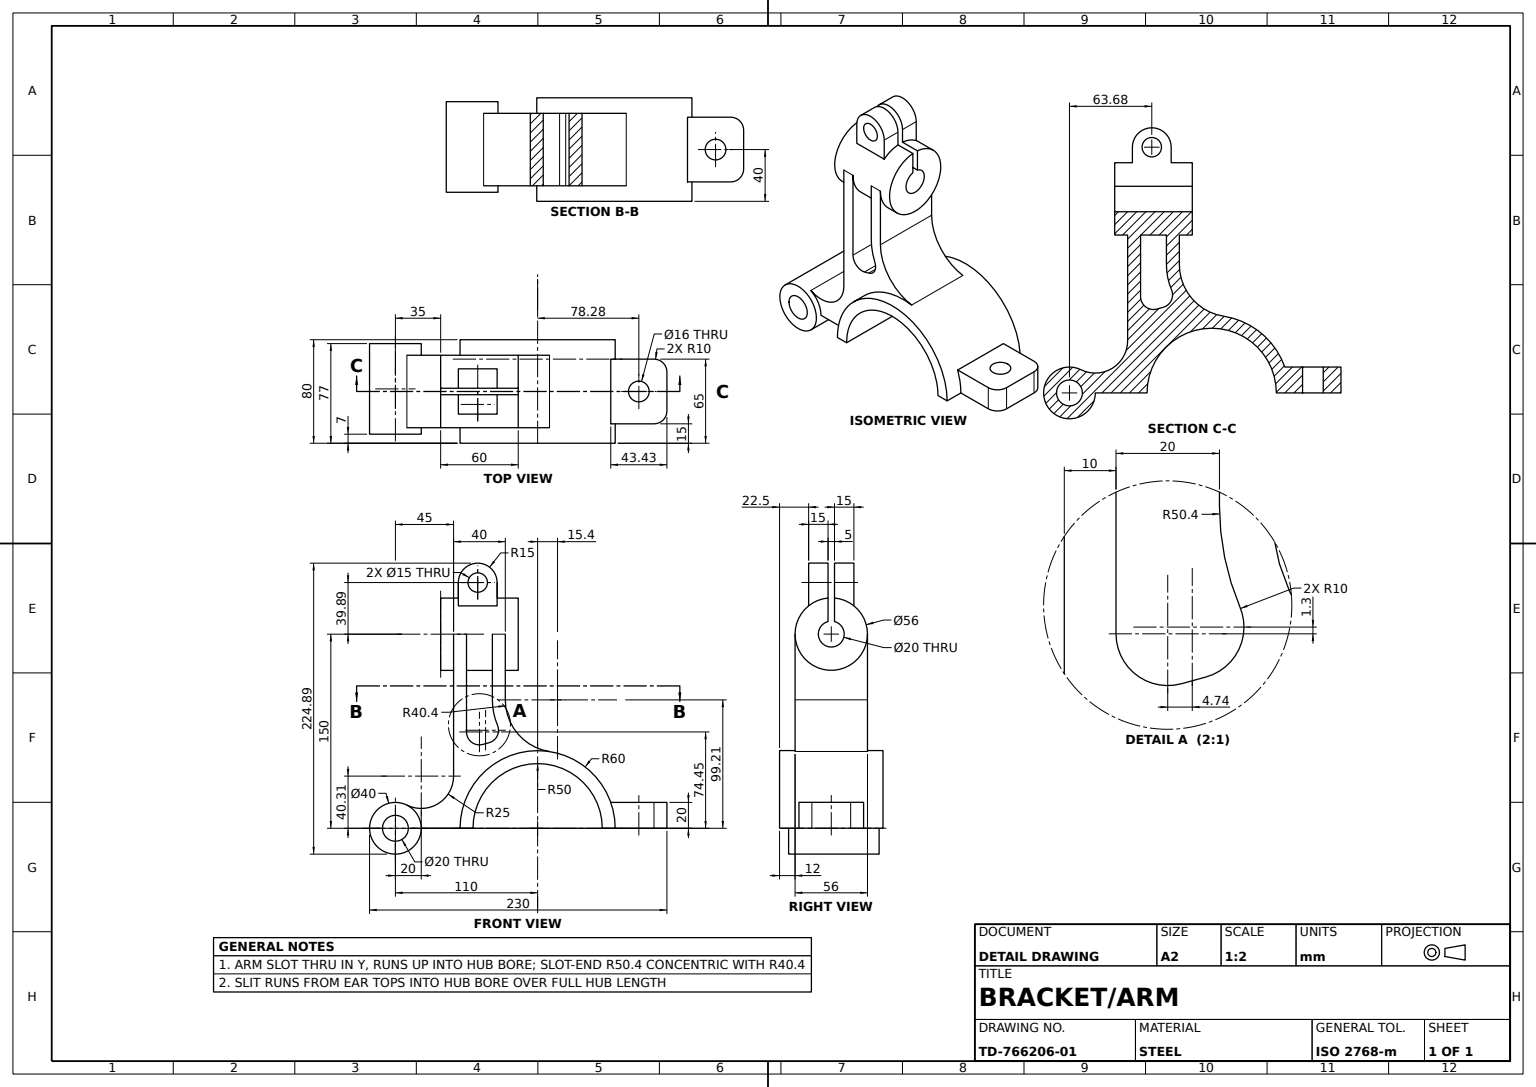
solid
v1 (-31.323438,177.88817,-2.5)
v2 (-31.323438,189.88817,-2.5)
e1 v1 v2 LINE
v3 (-61.323438,189.88817,-2.5)
e2 v2 v3 CIRCLE(AX(P(-46.323438,189.88817,-2.5),D(0,0,1),D(1,0,0)),15)
v4 (-61.323438,177.88817,-2.5)
e3 v3 v4 LINE
v5 (-75,177.88817,-2.5)
e4 v4 v5 LINE
v6 (-75,159.682458,-2.5)
e5 v5 v6 LINE
v7 (-15,159.682458,-2.5)
e6 v7 v6 LINE
v8 (-15,177.88817,-2.5)
e7 v7 v8 LINE
e8 v8 v1 LINE
v9 (-53.823438,189.88817,-2.5)
v10 (-38.823438,189.88817,-2.5)
e9 v9 v10 CIRCLE(AX(P(-46.323438,189.88817,-2.5),D(0,0,-1),D(-1,0,0)),7.5)
e10 v10 v9 CIRCLE(AX(P(-46.323438,189.88817,-2.5),D(0,0,-1),D(-1,0,0)),7.5)
face PLANE(AX(P(26,0,-2.5),D(0,0,-1),D(-1,0,0))) rev [e1 e2 e3 e4 e5 -e6 e7 e8] [e9 e10]
v11 (50,0,-40)
v12 (60,0,-40)
e11 v11 v12 LINE
v13 (-50,0,-40)
e12 v13 v11 CIRCLE(AX(P(0,0,-40),D(0,0,-1),D(1,0,0)),50)
v14 (-60,0,-40)
e13 v14 v13 LINE
e14 v12 v14 CIRCLE(AX(P(0,0,-40),D(0,0,1),D(1,0,0)),60)
face PLANE(AX(P(0,0,-40),D(0,0,1),D(1,0,0))) rev [-e11 -e12 -e13 -e14]
v15 (-130,0,-37)
v16 (-90,0,-37)
e15 v15 v16 CIRCLE(AX(P(-110,0,-37),D(0,0,1),D(1,0,0)),20)
v17 (-90,0,-28)
e16 v16 v17 LINE
v18 (-90,0,28)
e17 v17 v18 LINE
v19 (-90,0,33)
e18 v18 v19 LINE
v20 (-130,0,33)
e19 v20 v19 CIRCLE(AX(P(-110,0,33),D(0,0,1),D(1,0,0)),20)
e20 v15 v20 LINE
face CYL(AX(P(-110,0,-37),D(0,0,1),D(1,0,0)),20) [e15 e16 e17 e18 -e19 -e20]
v21 (-38.823438,189.88817,-17.5)
e21 v21 v10 LINE
v22 (-53.823438,189.88817,-17.5)
e22 v22 v9 LINE
e23 v21 v22 CIRCLE(AX(P(-46.323438,189.88817,-17.5),D(0,0,1),D(1,0,0)),7.5)
face CYL(AX(P(-46.323438,189.88817,-71.5),D(0,0,1),D(1,0,0)),7.5) rev [e21 -e9 -e22 -e23]
v23 (60,0,40)
v24 (-60,0,40)
e24 v23 v24 CIRCLE(AX(P(0,0,40),D(0,0,1),D(1,0,0)),60)
v25 (-50,0,40)
e25 v24 v25 LINE
v26 (50,0,40)
e26 v25 v26 CIRCLE(AX(P(0,0,40),D(0,0,-1),D(1,0,0)),50)
e27 v26 v23 LINE
face PLANE(AX(P(0,0,40),D(0,0,1),D(1,0,0))) [e24 e25 e26 e27]
v27 (-55,150,28)
v28 (-55,74.446056,28)
e28 v27 v28 LINE
v29 (-55,74.446056,-28)
e29 v29 v28 LINE
v30 (-55,150,-28)
e30 v30 v29 LINE
e31 v30 v27 CIRCLE(AX(P(-55,150,0),D(-1,0,0),D(0,0,1)),28)
face PLANE(AX(P(-55,0,-28),D(-1,0,0),D(0,0,1))) rev [e28 -e29 -e30 e31]
v31 (100,20,15)
v32 (90,20,25)
e32 v31 v32 CIRCLE(AX(P(90,20,15),D(0,-1,0),D(0,0,-1)),10)
v33 (90,0,25)
e33 v32 v33 LINE
v34 (100,0,15)
e34 v34 v33 CIRCLE(AX(P(90,0,15),D(0,-1,0),D(0,0,-1)),10)
e35 v31 v34 LINE
face CYL(AX(P(90,20,15),D(0,-1,0),D(0,0,-1)),10) [e32 e33 -e34 -e35]
v35 (90,0,-25)
v36 (100,0,-15)
e36 v35 v36 CIRCLE(AX(P(90,0,-15),D(0,-1,0),D(0,0,-1)),10)
e37 v36 v34 LINE
v37 (60,0,25)
e38 v33 v37 LINE
e39 v37 v23 LINE
e40 v11 v26 LINE
v38 (60,0,-25)
e41 v12 v38 LINE
e42 v38 v35 LINE
v39 (78.284271,0,-8)
v40 (78.284271,0,8)
e43 v39 v40 CIRCLE(AX(P(78.284271,0,0),D(0,-1,0),D(0,0,-1)),8)
e44 v40 v39 CIRCLE(AX(P(78.284271,0,0),D(0,-1,0),D(0,0,-1)),8)
face PLANE(AX(P(50,0,-40),D(0,-1,0),D(0,0,-1))) [e36 e37 e34 e38 e39 -e27 -e40 e11 e41 e42] [-e43 -e44]
e45 v19 v20 CIRCLE(AX(P(-110,0,33),D(0,0,1),D(1,0,0)),20)
v41 (-101.111111,17.916128,28)
e46 v18 v41 CIRCLE(AX(P(-110,0,28),D(0,0,1),D(1,0,0)),20)
v42 (-101.111111,17.916128,-28)
e47 v42 v41 LINE
e48 v17 v42 CIRCLE(AX(P(-110,0,-28),D(0,0,1),D(1,0,0)),20)
e49 v16 v15 CIRCLE(AX(P(-110,0,-37),D(0,0,1),D(1,0,0)),20)
face CYL(AX(P(-110,0,-37),D(0,0,1),D(1,0,0)),20) [-e45 -e18 e46 -e47 -e48 -e16 e49 e20]
v43 (-25,99.211169,-28)
v44 (9.202759,59.290043,-28)
e50 v43 v44 CIRCLE(AX(P(15.399153,99.211169,-28),D(0,0,1),D(1,0,0)),40.399153)
v45 (-25,99.211169,28)
e51 v43 v45 LINE
v46 (9.202759,59.290043,28)
e52 v45 v46 CIRCLE(AX(P(15.399153,99.211169,28),D(0,0,1),D(1,0,0)),40.399153)
e53 v44 v46 LINE
face CYL(AX(P(15.399153,99.211169,-28),D(0,0,1),D(1,0,0)),40.399153) rev [-e50 e51 e52 -e53]
v47 (-35,99.211169,-28)
v48 (-35,99.211169,28)
e54 v47 v48 LINE
v49 (-31.041399,79.631849,-28)
e55 v47 v49 CIRCLE(AX(P(15.399153,99.211169,-28),D(0,0,1),D(1,0,0)),50.399153)
v50 (-31.041399,79.631849,28)
e56 v49 v50 LINE
e57 v48 v50 CIRCLE(AX(P(15.399153,99.211169,28),D(0,0,1),D(1,0,0)),50.399153)
face CYL(AX(P(15.399153,99.211169,-28),D(0,0,1),D(1,0,0)),50.399153) [-e54 e55 e56 -e57]
v51 (-75,150,10)
v52 (-75,159.682458,2.5)
e58 v51 v52 CIRCLE(AX(P(-75,150,0),D(-1,0,0),D(0,0,1)),10)
v53 (-15,159.682458,2.5)
e59 v53 v52 LINE
v54 (-15,150,10)
e60 v53 v54 CIRCLE(AX(P(-15,150,0),D(1,0,0),D(0,0,-1)),10)
e61 v54 v51 LINE
face CYL(AX(P(26,150,0),D(-1,0,0),D(0,0,1)),10) rev [e58 -e59 e60 e61]
v55 (-31.323438,171.857493,-17.5)
e62 v1 v55 CIRCLE(AX(P(-31.323438,150,0),D(-1,0,0),D(0,0,-1)),28)
v56 (-31.323438,189.88817,-17.5)
e63 v55 v56 LINE
e64 v56 v2 LINE
face PLANE(AX(P(-31.323438,189.88817,-17.5),D(1,0,0),D(0,0,-1))) [e62 e63 e64 -e1]
v57 (-61.323438,171.857493,-17.5)
e65 v57 v55 LINE
v58 (-61.323438,189.88817,-17.5)
e66 v58 v57 LINE
e67 v56 v58 CIRCLE(AX(P(-46.323438,189.88817,-17.5),D(0,0,1),D(1,0,0)),15)
e68 v22 v21 CIRCLE(AX(P(-46.323438,189.88817,-17.5),D(0,0,1),D(1,0,0)),7.5)
face PLANE(AX(P(-46.323438,189.88817,-17.5),D(0,0,1),D(1,0,0))) rev [-e65 -e66 -e67 -e63] [e23 e68]
v59 (-35,150,-28)
e69 v30 v59 LINE
v60 (-35,150,28)
e70 v59 v60 CIRCLE(AX(P(-35,150,0),D(-1,0,0),D(0,0,1)),28)
e71 v27 v60 LINE
face CYL(AX(P(-75,150,0),D(1,0,0),D(0,0,-1)),28) [e69 e70 -e71 -e31]
v61 (-25,150,-28)
v62 (-25,150,28)
e72 v61 v62 CIRCLE(AX(P(-25,150,0),D(-1,0,0),D(0,0,1)),28)
v63 (-15,150,-28)
e73 v61 v63 LINE
v64 (-15,150,28)
e74 v64 v63 CIRCLE(AX(P(-15,150,0),D(1,0,0),D(0,0,-1)),28)
e75 v62 v64 LINE
face CYL(AX(P(-75,150,0),D(1,0,0),D(0,0,-1)),28) [-e72 e73 -e74 -e75]
e76 v58 v3 LINE
face CYL(AX(P(-46.323438,189.88817,-17.5),D(0,0,1),D(1,0,0)),15) [e76 -e2 -e64 e67]
face CYL(AX(P(-46.323438,189.88817,-71.5),D(0,0,1),D(1,0,0)),7.5) rev [-e10 -e21 -e68 e22]
v65 (100,20,-15)
e77 v65 v36 LINE
e78 v65 v31 LINE
face PLANE(AX(P(100,20,0),D(1,0,0),D(0,0,-1))) [-e77 e78 e35 -e37]
v66 (-53.823438,189.88817,17.5)
v67 (-38.823438,189.88817,17.5)
e79 v66 v67 CIRCLE(AX(P(-46.323438,189.88817,17.5),D(0,0,1),D(1,0,0)),7.5)
e80 v67 v66 CIRCLE(AX(P(-46.323438,189.88817,17.5),D(0,0,1),D(1,0,0)),7.5)
v68 (-31.323438,189.88817,17.5)
v69 (-61.323438,189.88817,17.5)
e81 v68 v69 CIRCLE(AX(P(-46.323438,189.88817,17.5),D(0,0,1),D(1,0,0)),15)
v70 (-61.323438,171.857493,17.5)
e82 v69 v70 LINE
v71 (-31.323438,171.857493,17.5)
e83 v71 v70 LINE
e84 v71 v68 LINE
face PLANE(AX(P(-46.323438,189.88817,17.5),D(0,0,-1),D(1,0,0))) rev [-e79 -e80] [e81 e82 -e83 e84]
v72 (78.284271,20,-8)
v73 (78.284271,20,8)
e85 v72 v73 CIRCLE(AX(P(78.284271,20,0),D(0,1,0),D(0,0,1)),8)
e86 v40 v73 LINE
e87 v39 v72 LINE
face CYL(AX(P(78.284271,-25,0),D(0,1,0),D(0,0,1)),8) rev [e85 -e86 e44 e87]
e88 v13 v25 LINE
face CYL(AX(P(0,0,-40),D(0,0,1),D(1,0,0)),50) rev [-e26 -e88 e12 e40]
v74 (-65,150,-28)
v75 (-65,150,28)
e89 v74 v75 CIRCLE(AX(P(-65,150,0),D(-1,0,0),D(0,0,1)),28)
v76 (-65,40.311289,-28)
e90 v74 v76 LINE
v77 (-65,40.311289,28)
e91 v76 v77 LINE
e92 v75 v77 LINE
face PLANE(AX(P(-65,0,-28),D(-1,0,0),D(0,0,1))) [-e89 e90 e91 -e92]
v78 (-60,0,-28)
e93 v78 v17 LINE
e94 v14 v78 LINE
v79 (-60,0,28)
e95 v79 v24 LINE
e96 v79 v18 LINE
face PLANE(AX(P(-60,0,-40),D(0,-1,0),D(0,0,-1))) [-e93 -e94 e13 e88 -e25 -e95 e96 -e17]
v80 (-75,150,28)
v81 (-75,150,-28)
e97 v80 v81 CIRCLE(AX(P(-75,150,0),D(1,0,0),D(0,0,-1)),28)
e98 v81 v74 LINE
e99 v80 v75 LINE
face CYL(AX(P(-75,150,0),D(1,0,0),D(0,0,-1)),28) [e97 e98 e89 -e99]
v82 (90,20,-25)
e100 v82 v35 LINE
e101 v82 v65 CIRCLE(AX(P(90,20,-15),D(0,-1,0),D(0,0,-1)),10)
face CYL(AX(P(90,20,-15),D(0,-1,0),D(0,0,-1)),10) [-e100 e101 e77 -e36]
v83 (-75,150,-10)
e102 v83 v51 CIRCLE(AX(P(-75,150,0),D(-1,0,0),D(0,0,1)),10)
e103 v6 v83 CIRCLE(AX(P(-75,150,0),D(-1,0,0),D(0,0,1)),10)
e104 v81 v5 CIRCLE(AX(P(-75,150,0),D(1,0,0),D(0,0,-1)),28)
v84 (-75,177.88817,2.5)
e105 v84 v80 CIRCLE(AX(P(-75,150,0),D(1,0,0),D(0,0,-1)),28)
e106 v52 v84 LINE
face PLANE(AX(P(-75,150,0),D(1,0,0),D(0,0,-1))) rev [-e102 -e103 -e5 -e104 -e97 -e105 -e106 -e58]
e107 v75 v27 LINE
e108 v60 v62 LINE
v85 (-15,177.88817,2.5)
e109 v85 v64 CIRCLE(AX(P(-15,150,0),D(1,0,0),D(0,0,-1)),28)
v86 (-31.323438,177.88817,2.5)
e110 v85 v86 LINE
e111 v86 v71 CIRCLE(AX(P(-31.323438,150,0),D(1,0,0),D(0,-1,0)),28)
v87 (-61.323438,177.88817,2.5)
e112 v70 v87 CIRCLE(AX(P(-61.323438,150,0),D(-1,0,0),D(0,0,-1)),28)
e113 v87 v84 LINE
face CYL(AX(P(-75,150,0),D(1,0,0),D(0,0,-1)),28) [e107 e71 e108 e75 -e109 e110 e111 e83 e112 e113 e105 e99]
e114 v62 v45 LINE
e115 v60 v48 LINE
v88 (-30.255949,75.746998,28)
e116 v88 v50 CIRCLE(AX(P(-40.255949,75.746998,28),D(0,0,1),D(1,0,0)),10)
v89 (-37.611325,66.103038,28)
e117 v89 v88 CIRCLE(AX(P(-40.255949,75.746998,28),D(0,0,1),D(1,0,0)),10)
v90 (-42.355377,64.802096,28)
e118 v90 v89 LINE
e119 v28 v90 CIRCLE(AX(P(-45,74.446056,28),D(0,0,1),D(1,0,0)),10)
e120 v41 v77 CIRCLE(AX(P(-90,40.311289,28),D(0,0,1),D(1,0,0)),25)
e121 v46 v79 CIRCLE(AX(P(0,0,28),D(0,0,1),D(1,0,0)),60)
face PLANE(AX(P(0,0,28),D(0,0,1),D(1,0,0))) [-e52 -e114 -e108 e115 e57 -e116 -e117 -e118 -e119 -e28 -e107 e92 -e120 -e46 -e96 -e121]
e122 v59 v47 LINE
face PLANE(AX(P(-35,0,-28),D(-1,0,0),D(0,0,1))) [-e70 e122 e54 -e115]
v91 (-42.355377,64.802096,-28)
e123 v91 v90 LINE
e124 v29 v91 CIRCLE(AX(P(-45,74.446056,-28),D(0,0,1),D(1,0,0)),10)
face CYL(AX(P(-45,74.446056,-28),D(0,0,1),D(1,0,0)),10) rev [e29 e119 -e123 -e124]
v92 (56.568542,20,-25)
e125 v38 v92 CIRCLE(AX(P(0,0,-25),D(0,0,1),D(-1,0,0)),60)
e126 v92 v82 LINE
face PLANE(AX(P(50,20,-25),D(0,0,-1),D(-1,0,0))) [e125 e126 e100 -e42]
v93 (-61.323438,189.88817,2.5)
e127 v93 v87 LINE
v94 (-31.323438,189.88817,2.5)
e128 v94 v93 CIRCLE(AX(P(-46.323438,189.88817,2.5),D(0,0,1),D(1,0,0)),15)
e129 v86 v94 LINE
e130 v85 v53 LINE
v95 (-38.823438,189.88817,2.5)
v96 (-53.823438,189.88817,2.5)
e131 v95 v96 CIRCLE(AX(P(-46.323438,189.88817,2.5),D(0,0,1),D(1,0,0)),7.5)
e132 v96 v95 CIRCLE(AX(P(-46.323438,189.88817,2.5),D(0,0,1),D(1,0,0)),7.5)
face PLANE(AX(P(26,0,2.5),D(0,0,1),D(1,0,0))) rev [-e113 -e127 -e128 -e129 -e110 e130 e59 e106] [e131 e132]
v97 (-100,0,33)
v98 (-120,0,33)
e133 v97 v98 CIRCLE(AX(P(-110,0,33),D(0,0,1),D(1,0,0)),10)
e134 v98 v97 CIRCLE(AX(P(-110,0,33),D(0,0,1),D(1,0,0)),10)
face PLANE(AX(P(-110,0,33),D(0,0,1),D(1,0,0))) [e19 e45] [-e133 -e134]
e135 v68 v94 LINE
face PLANE(AX(P(-31.323438,177.88817,17.5),D(-1,0,0),D(0,-1,0))) rev [-e135 -e84 -e111 e129]
v99 (-37.611325,66.103038,-28)
e136 v99 v89 LINE
e137 v91 v99 LINE
face PLANE(AX(P(-19.489892,71.072403,-28),D(0.264462342,-0.964396013,0),D(0.964396013,0.264462342,0))) rev [e118 -e136 -e137 e123]
v100 (-120,0,-37)
v101 (-100,0,-37)
e138 v100 v101 CIRCLE(AX(P(-110,0,-37),D(0,0,1),D(1,0,0)),10)
e139 v101 v100 CIRCLE(AX(P(-110,0,-37),D(0,0,1),D(1,0,0)),10)
face PLANE(AX(P(-110,0,-37),D(0,0,1),D(1,0,0))) rev [-e49 -e15] [e138 e139]
v102 (-15,150,-10)
e140 v54 v102 CIRCLE(AX(P(-15,150,0),D(1,0,0),D(0,0,-1)),10)
e141 v102 v83 LINE
face CYL(AX(P(26,150,0),D(-1,0,0),D(0,0,1)),10) rev [e102 -e61 e140 e141]
e142 v73 v72 CIRCLE(AX(P(78.284271,20,0),D(0,1,0),D(0,0,1)),8)
face CYL(AX(P(78.284271,-25,0),D(0,1,0),D(0,0,1)),8) rev [e142 -e87 e43 e86]
v103 (-30.255949,75.746998,-28)
e143 v103 v49 CIRCLE(AX(P(-40.255949,75.746998,-28),D(0,0,1),D(1,0,0)),10)
e144 v103 v88 LINE
face CYL(AX(P(-40.255949,75.746998,-28),D(0,0,1),D(1,0,0)),10) rev [e116 -e56 -e143 e144]
e145 v101 v97 LINE
e146 v100 v98 LINE
face CYL(AX(P(-110,0,-56),D(0,0,1),D(1,0,0)),10) rev [e145 e133 -e146 -e139]
e147 v102 v7 CIRCLE(AX(P(-15,150,0),D(1,0,0),D(0,0,-1)),10)
e148 v63 v8 CIRCLE(AX(P(-15,150,0),D(1,0,0),D(0,0,-1)),28)
face PLANE(AX(P(-15,150,0),D(1,0,0),D(0,0,-1))) [-e147 -e140 -e60 -e130 e109 e74 e148 -e7]
e149 v57 v4 CIRCLE(AX(P(-61.323438,150,0),D(1,0,0),D(0,0,1)),28)
face PLANE(AX(P(-61.323438,177.88817,-17.5),D(-1,0,0),D(0,0,1))) [e66 e149 -e3 -e76]
face CYL(AX(P(-110,0,-56),D(0,0,1),D(1,0,0)),10) rev [e134 -e145 -e138 e146]
e150 v61 v43 LINE
face PLANE(AX(P(-25,0,-28),D(-1,0,0),D(0,0,1))) rev [e114 -e51 -e150 e72]
v104 (56.568542,20,25)
e151 v104 v92 LINE
e152 v32 v104 LINE
face PLANE(AX(P(90,20,-15),D(0,-1,0),D(0,0,-1))) rev [-e126 -e151 -e152 -e32 -e78 -e101] [-e142 -e85]
e153 v42 v76 CIRCLE(AX(P(-90,40.311289,-28),D(0,0,1),D(1,0,0)),25)
face CYL(AX(P(-90,40.311289,-28),D(0,0,1),D(1,0,0)),25) rev [e120 -e91 -e153 e47]
face CYL(AX(P(26,150,0),D(-1,0,0),D(0,0,1)),10) rev [e147 e6 e103 -e141]
e154 v69 v93 LINE
face PLANE(AX(P(-61.323438,177.88817,17.5),D(1,0,0),D(0,0,-1))) rev [-e82 e154 e127 -e112]
e155 v59 v61 LINE
e156 v74 v30 LINE
face CYL(AX(P(-75,150,0),D(1,0,0),D(0,0,-1)),28) [-e149 e65 -e62 -e8 -e148 -e73 -e155 -e69 -e156 -e98 e104 -e4]
e157 v44 v78 CIRCLE(AX(P(0,0,-28),D(0,0,1),D(1,0,0)),60)
e158 v104 v37 CIRCLE(AX(P(0,0,25),D(0,0,-1),D(1,0,0)),60)
face CYL(AX(P(0,0,-40),D(0,0,1),D(1,0,0)),60) [e94 -e157 e53 e121 e95 -e24 -e39 -e158 e151 -e125 -e41 e14]
e159 v95 v67 LINE
e160 v96 v66 LINE
face CYL(AX(P(-46.323438,189.88817,-71.5),D(0,0,1),D(1,0,0)),7.5) rev [-e131 e159 e80 -e160]
face CYL(AX(P(-46.323438,189.88817,-71.5),D(0,0,1),D(1,0,0)),7.5) rev [-e132 e160 e79 -e159]
face CYL(AX(P(-46.323438,189.88817,17.5),D(0,0,-1),D(-1,0,0)),15) [e135 e128 -e154 -e81]
e161 v99 v103 CIRCLE(AX(P(-40.255949,75.746998,-28),D(0,0,1),D(1,0,0)),10)
face PLANE(AX(P(0,0,-28),D(0,0,1),D(1,0,0))) rev [e124 e137 e161 e143 -e55 -e122 e155 e150 e50 e157 e93 e48 e153 -e90 e156 e30]
face CYL(AX(P(-40.255949,75.746998,-28),D(0,0,1),D(1,0,0)),10) rev [-e161 e136 e117 -e144]
face PLANE(AX(P(90,20,25),D(0,0,1),D(1,0,0))) [e158 -e38 -e33 e152]
